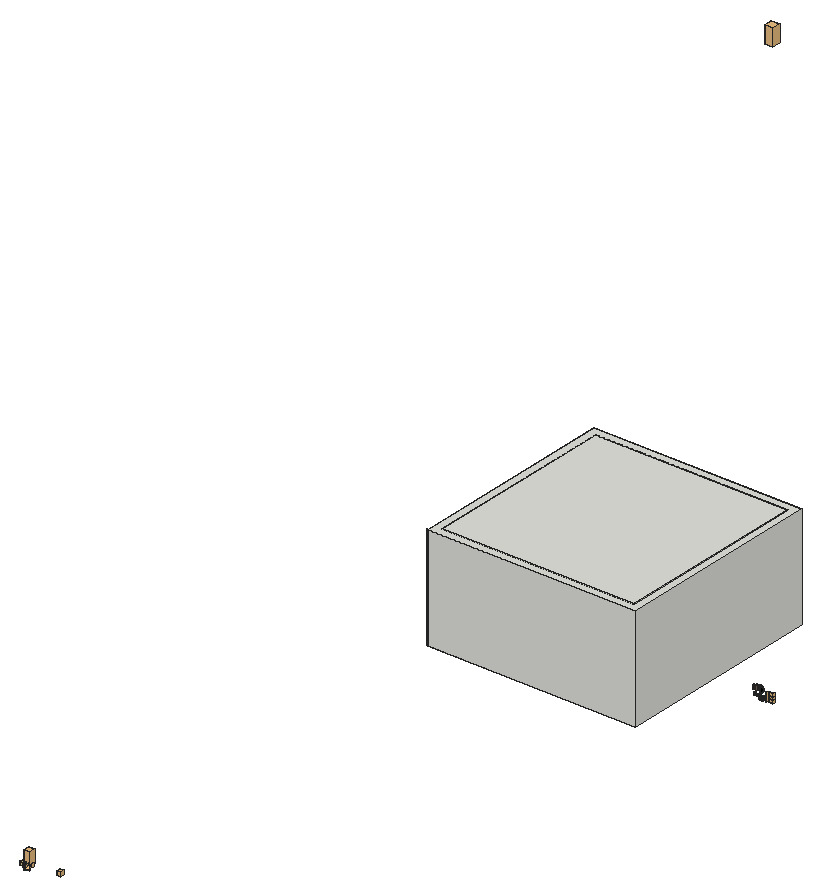
# SketchUp Ruby script. Lengths in inches.
U = 1.inch
M = Sketchup.active_model
def pt(a) = Geom::Point3d.new(a.map { |v| v * U })
def face(e, loops, mat)
  f = e.add_face(loops[0].map { |a| pt(a) })
  loops[1..].each { |l| e.add_face(l.map { |a| pt(a) }).erase! }
  f.material = f.back_material = mat if mat
  f
end
# faces: each face lists its corners as indices into pts; further lists are holes
def faces(e, pts, list, mat = nil) = list.each { |f| face(e, (f[0].is_a?(Array) ? f : [f]).map { |l| l.map { |i| pts[i] } }, mat) }
# xy, xz, yz: faces in a plane at the given z, y or x. An outline is a flat list of corners, or four numbers for a rectangle; further outlines are holes
def ring(l) = l.size == 4 ? [[l[0], l[1]], [l[2], l[1]], [l[2], l[3]], [l[0], l[3]]] : l.each_slice(2).to_a
def flat(e, list, mat, &to3) = list.each { |f| face(e, (f[0].is_a?(Array) ? f : [f]).map { |l| ring(l).map { |u, v| to3.(u, v) } }, mat) }
def xy(e, z, list, mat = nil) = flat(e, list, mat) { |x, y| [x, y, z] }
def xz(e, y, list, mat = nil) = flat(e, list, mat) { |x, z| [x, y, z] }
def yz(e, x, list, mat = nil) = flat(e, list, mat) { |y, z| [x, y, z] }
def lines(e, pts, list) = list.each { |a, b| e.add_line(pt(pts[a]), pt(pts[b])) }
# prism: a flat outline (further loops are holes) pulled along v
def prism(e, loops, v, mat = nil)
  f = face(e, loops, mat); d = Geom::Vector3d.new(v.map { |x| x * U })
  f.pushpull(f.normal.samedirection?(d) ? d.length : -d.length)
end
def box(e, o, s, mat = nil) = prism(e, [[o, [o[0] + s[0], o[1], o[2]], [o[0] + s[0], o[1] + s[1], o[2]], [o[0], o[1] + s[1], o[2]]]], [0, 0, s[2]], mat)
def at(x, y, z, deg = 0) = Geom::Transformation.translation(pt([x, y, z])) * Geom::Transformation.rotation(ORIGIN, Z_AXIS, deg.degrees)
def axes(o, x, y, z) = Geom::Transformation.new([*x, 0, *y, 0, *z, 0, *pt(o).to_a, 1])
def part(name) = M.definitions.add(name)
# library, detail: a bought-in or finely detailed component or shape, given as its bounding box
def library(name, o, s) = part(name).tap { |d| box(d.entities, o, s) }
def detail(e, o, s) = box(e.add_group.entities, o, s)
def put(e, d, t, mat = nil) = e.add_instance(d, t).tap { |i| i.material = mat if mat }
def group(e, t, mat = nil) = e.add_group.tap { |g| g.transformation = t; g.material = mat if mat }.entities
root = M.entities
M.materials.add("Lily_Light").color = [246, 247, 58]
M.materials.add("Polytec Natio Walnut").color = [132, 104, 79]
M.materials.add("SAMSUNG SMART FRIDGE").color = [78, 78, 81]
M.materials.add("[0045_Goldenrod]").color = [218, 165, 31]
M.materials["[0045_Goldenrod]"].alpha = 0.63
M.materials.add("[0066_Honeydew]").color = [240, 255, 240]
M.materials.add("[0130_Gainsboro]").color = [219, 219, 219]
M.materials.add("[0133_Gray]").color = [63, 63, 63]
M.materials.add("[Color M09]4").color = [0, 0, 0]
M.materials.add("[Translucent Glass Blue]").color = [100, 149, 237]
M.materials["[Translucent Glass Blue]"].alpha = 0.5
M.materials.add("cnwhc.com_草图联盟_1kmauOsh").color = [54, 52, 52]
M.materials.add("cnwhc.com_草图联盟_C8Y5Xp2O").color = [156, 156, 156]
M.materials["cnwhc.com_草图联盟_C8Y5Xp2O"].alpha = 0.15
M.materials.add("cnwhc.com_草图联盟_IHFcDxe1").color = [138, 151, 59]
M.materials.add("cnwhc.com_草图联盟_KNEfX85g").color = [162, 126, 87]
M.materials.add("cnwhc.com_草图联盟_QJow1Ky4").color = [144, 133, 65]
M.materials.add("cnwhc.com_草图联盟_z6N5x4Hv").color = [223, 205, 124]
c1 = part("Door Lever\#2")
detail(c1.entities,[0,0,0],[5.43,2.05,2.36])
c2 = part("Door Lever\#1")
detail(c2.entities,[0,0,0],[5.43,2.05,2.36])
c3 = part("Door Lever\#3")
detail(c3.entities,[0,0,0],[5.43,2.05,2.36])
c4 = part("200mm Half Round Handle")
xz(c4.entities,0,[[3.9375,0,3.9375,7.875,3.42,7.84,2.92,7.74,2.43,7.57,1.97,7.35,1.54,7.06,1.15,6.72,0.8125,6.33,0.53,5.91,0.3,5.44,0.13,4.96,0.03,4.45,0,3.9375,0.03,3.42,0.13,2.92,0.3,2.43,0.53,1.97,0.8125,1.54,1.15,1.15,1.54,0.8125,1.97,0.53,2.43,0.3,2.92,0.13,3.42,0.03]],"[Color M09]4")
xz(c4.entities,0.12,[[3.82,0.01,3.42,0.03,2.92,0.13,2.43,0.3,1.97,0.53,1.54,0.8125,1.15,1.15,0.8125,1.54,0.53,1.97,0.3,2.43,0.13,2.92,0.03,3.42,0,3.9375,0.03,4.45,0.13,4.96,0.3,5.44,0.53,5.91,0.8125,6.33,1.15,6.72,1.54,7.06,1.97,7.35,2.43,7.57,2.92,7.74,3.42,7.84,3.82,7.87]],"[Color M09]4")
xz(c4.entities,0.91,[[3.9375,0,3.82,0.01,3.82,7.87,3.9375,7.875]],"[Color M09]4")
yz(c4.entities,3.82,[[0.12,0.01,0.91,7.87]],"[Color M09]4")
yz(c4.entities,3.9375,[[0,0,0.91,7.875]],"[Color M09]4")
p = [[3.42,0,0.03],[2.92,0,0.13],[2.92,0.12,0.13],[3.42,0.12,0.03],[3.9375,0,0],[3.82,0.12,0.01],
  [3.82,0.91,0.01],[3.9375,0.91,0],[2.43,0,0.3],[2.43,0.12,0.3],[1.97,0,0.53],[1.97,0.12,0.53],
  [1.54,0,0.8125],[1.54,0.12,0.8125],[1.15,0,1.15],[1.15,0.12,1.15],[0.8125,0,1.54],[0.8125,0.12,1.54],
  [0.53,0,1.97],[0.53,0.12,1.97],[0.3,0,2.43],[0.3,0.12,2.43],[0.13,0,2.92],[0.13,0.12,2.92],
  [0.03,0,3.42],[0.03,0.12,3.42],[0,0,3.9375],[0,0.12,3.9375],[0.03,0,4.45],[0.03,0.12,4.45],
  [0.13,0,4.96],[0.13,0.12,4.96],[0.3,0,5.44],[0.3,0.12,5.44],[0.53,0,5.91],[0.53,0.12,5.91],
  [0.8125,0,6.33],[0.8125,0.12,6.33],[1.15,0,6.72],[1.15,0.12,6.72],[1.54,0,7.06],[1.54,0.12,7.06],
  [1.97,0,7.35],[1.97,0.12,7.35],[2.43,0,7.57],[2.43,0.12,7.57],[2.92,0,7.74],[2.92,0.12,7.74],
  [3.42,0,7.84],[3.42,0.12,7.84],[3.9375,0,7.875],[3.9375,0.91,7.875],[3.82,0.91,7.87],[3.82,0.12,7.87]]
faces(c4.entities,p,[[0,1,2,3],[4,0,3,5,6,7],[1,8,9,2],[8,10,11,9],[10,12,13,11],[12,14,15,13],[14,16,17,15],[16,18,19,17],
  [18,20,21,19],[20,22,23,21],[22,24,25,23],[24,26,27,25],[26,28,29,27],[28,30,31,29],[30,32,33,31],[32,34,35,33],
  [34,36,37,35],[36,38,39,37],[38,40,41,39],[40,42,43,41],[42,44,45,43],[44,46,47,45],[46,48,49,47],[48,50,51,52,53,49]],"[Color M09]4")
c5 = part("150mm Half Round Handle")
xz(c5.entities,0,[[0,0,0.12,0.01,0.12,5.9,0,5.91]],"Polytec Natio Walnut")
xz(c5.entities,0.79,[[0.12,0.01,0.39,0.03,0.76,0.1,1.13,0.22,1.48,0.4,1.8,0.61,2.09,0.86,2.34,1.16,2.56,1.48,2.73,1.82,2.85,2.1875,2.93,2.57,2.95,2.95,2.93,3.34,2.85,3.72,2.73,4.08,2.56,4.43,2.34,4.75,2.09,5.04,1.8,5.3,1.48,5.51,1.13,5.68,0.76,5.8,0.39,5.88,0.12,5.9]],"Polytec Natio Walnut")
xz(c5.entities,0.91,[[0,0,0,5.91,0.39,5.88,0.76,5.8,1.13,5.68,1.48,5.51,1.8,5.3,2.09,5.04,2.34,4.75,2.56,4.43,2.73,4.08,2.85,3.72,2.93,3.34,2.95,2.95,2.93,2.57,2.85,2.1875,2.73,1.82,2.56,1.48,2.34,1.16,2.09,0.86,1.8,0.61,1.48,0.4,1.13,0.22,0.76,0.1,0.39,0.03]],"Polytec Natio Walnut")
yz(c5.entities,0,[[0,0,0.91,5.91]],"Polytec Natio Walnut")
yz(c5.entities,0.12,[[0,0.01,0.79,5.9]],"Polytec Natio Walnut")
p = [[0,0.91,0],[0.39,0.91,0.03],[0.39,0.79,0.03],[0.12,0.79,0.01],[0.12,0,0.01],[0,0,0],
  [0.76,0.91,0.1],[0.76,0.79,0.1],[1.13,0.91,0.22],[1.13,0.79,0.22],[1.48,0.91,0.4],[1.48,0.79,0.4],
  [1.8,0.91,0.61],[1.8,0.79,0.61],[2.09,0.91,0.86],[2.09,0.79,0.86],[2.34,0.91,1.16],[2.34,0.79,1.16],
  [2.56,0.91,1.48],[2.56,0.79,1.48],[2.73,0.91,1.82],[2.73,0.79,1.82],[2.85,0.91,2.1875],[2.85,0.79,2.1875],
  [2.93,0.91,2.57],[2.93,0.79,2.57],[2.95,0.91,2.95],[2.95,0.79,2.95],[2.93,0.91,3.34],[2.93,0.79,3.34],
  [2.85,0.91,3.72],[2.85,0.79,3.72],[2.73,0.91,4.08],[2.73,0.79,4.08],[2.56,0.91,4.43],[2.56,0.79,4.43],
  [2.34,0.91,4.75],[2.34,0.79,4.75],[2.09,0.91,5.04],[2.09,0.79,5.04],[1.8,0.91,5.3],[1.8,0.79,5.3],
  [1.48,0.91,5.51],[1.48,0.79,5.51],[1.13,0.91,5.68],[1.13,0.79,5.68],[0.76,0.91,5.8],[0.76,0.79,5.8],
  [0.39,0.91,5.88],[0.39,0.79,5.88],[0,0.91,5.91],[0,0,5.91],[0.12,0,5.9],[0.12,0.79,5.9]]
faces(c5.entities,p,[[0,1,2,3,4,5],[1,6,7,2],[6,8,9,7],[8,10,11,9],[10,12,13,11],[12,14,15,13],[14,16,17,15],[16,18,19,17],
  [18,20,21,19],[20,22,23,21],[22,24,25,23],[24,26,27,25],[26,28,29,27],[28,30,31,29],[30,32,33,31],[32,34,35,33],
  [34,36,37,35],[36,38,39,37],[38,40,41,39],[40,42,43,41],[42,44,45,43],[44,46,47,45],[46,48,49,47],[48,50,51,52,53,49]],"Polytec Natio Walnut")
c6 = part("148mm Black Satin Pull\#1")
prism(c6.entities,[[[5.83,0.12,0.5],[5.83,0.16,0.49],[5.83,0.16,0],[5.83,0.31,0],[5.83,0.31,0.49],[5.83,0.35,0.5],[5.83,0.4,0.54],[5.83,0.44,0.59],[5.83,0.46,0.65],[5.83,0.47,0.71],[5.83,0.46,0.77],[5.83,0.44,0.83],[5.83,0.4,0.875],[5.83,0.35,0.91],[5.83,0.3,0.9375],[5.83,0.24,0.94],[5.83,0.18,0.9375],[5.83,0.12,0.91],[5.83,0.07,0.875],[5.83,0.03,0.83],[5.83,0.01,0.77],[5.83,0,0.71],[5.83,0.01,0.65],[5.83,0.03,0.59],[5.83,0.07,0.54]]],[-5.83,0,0],"[Color M09]4")
p = [[5.83,0.16,0.59],[0,0.16,0.59],[5.83,0.31,0.59],[0,0.31,0.59]]
lines(c6.entities,p,[[0,1],[2,3]])
c7 = part("232mm Slimline Handle\#1")
detail(c7.entities,[0,0,0],[9.13,0.47,1.38])
c8 = part("232mm Slimline Handle")
detail(c8.entities,[0,0,0],[9.13,0.47,1.38])
c9 = library("SAMSUNG SMART FRIDGE",[0,-0.09,0],[35.91,28.28,70.08])
c10 = library("Bosch Stove",[0,0,0],[36.22,20.12,1.38])
c11 = library("fff.dwg",[0.01,-0.93,0],[23.6,19.21,16.14])
c12 = part("Janela aluminio")
xy(c12.entities,0,[[0,0,47.24,1.57],[23.62,1.57,47.24,2.76],[0,2.76,25.98,3.9375],[0,3.9375,47.24,5.91]])
xy(c12.entities,43.31,[[0,0,47.24,1.57],[23.62,1.57,47.24,2.76],[0,2.76,0,5.91,47.24,5.91,47.24,3.9375,25.98,3.9375,25.98,2.76],[25.98,2.76,47.24,3.9375]])
xz(c12.entities,1.57,[[0,0,23.62,0,23.62,41.34,21.26,41.34,21.26,1.97,1.97,1.97,1.97,41.34,23.62,41.34,23.62,43.31,0,43.31],[[23.62,0,47.24,43.31],[25.7,1.97,45.28,41.34]]])
xz(c12.entities,2.76,[[[0,0,23.62,43.31],[2.36,2.36,21.26,40.94]],[23.62,0,25.98,43.31]])
xz(c12.entities,2.76,[[2.36,2.36,21.26,40.94]],"[Translucent Glass Blue]")
xz(c12.entities,3.9375,[[25.98,0,25.98,2.36,44.88,2.36,44.88,40.94,25.98,40.94,25.98,43.31,47.24,43.31,47.24,0]])
xz(c12.entities,3.9375,[[25.98,2.36,44.88,40.94]],"[Translucent Glass Blue]")
yz(c12.entities,0,[[0,0,1.57,43.31],[2.76,0,5.91,43.31]])
yz(c12.entities,23.62,[[1.57,0,2.76,43.31]])
yz(c12.entities,25.98,[[2.76,0,3.9375,43.31]])
yz(c12.entities,47.24,[[0,0,1.57,43.31],[1.57,0,2.76,43.31],[3.9375,0,5.91,43.31]])
c13 = library("Sink with faucet",[-0.11,0,0],[20.3,18.9,21.51])
c14 = library("Potted plant",[0.24,-1.94,0],[14.49,14.49,6.23])
c15 = library("KITCHEN+KNIFES",[-11.85,-0.97,-1.38],[30.4,24.23,12.79])
c16 = library("Micro+samsungCE170b-b+28L",[0.33,0.39,0],[20.66,20.36,12.2])
c17 = library("Lg+Water+purifier (1)",[0,2.4,0],[10.83,14.37,19.92])
c18 = library("Group8",[-17.72,-4.29,0],[35.44,8.58,13.65])
c19 = library("Group\#13",[-397.46,82.38,-0.11],[62.88,62.86,260])
c20 = library("Group\#10",[-282.65,82.375,-0.11],[62.85,62.875,260.02])
c21 = library("Group\#9",[222.96,189.98,-0.44],[259.48,39.25,337.49])
c22 = library("Group\#30",[41.52,-158.49,40.25],[95.93,90.14,172.87])
c23 = library("Group\#21",[-504.125,120.57,-0.1],[108.2,108.21,338.13])
c24 = library("Group\#22",[-376.9,120.94,-0.1],[107.79,107.8,326.37])
c25 = library("Group\#8",[-254.81,120.48,-0.6],[108.21,108.21,334.5])
c26 = library("Group\#24",[-133.01,121.19,-0.1],[106.95,106.95,324.89])
c27 = library("Group\#25",[0.46,121.12,-0.1],[106.94,106.94,338.14])
c28 = library("Group\#26",[151.35,137.54,-0.1],[70.51,70.14,256.45])
c29 = library("Group\#27",[-266.02,-201.27,40.23],[225.02,228.69,89.38])
c30 = library("Group\#7",[-78.56,-74.98,40.25],[131.28,107.59,245.3125])
c31 = library("Group\#31",[-60.55,-181.2,40.41],[105.85,106.35,65.49])
c32 = library("Group\#34",[253.59,42.68,151.97],[53.13,53.13,100.94])
c33 = library("Group\#35",[281.12,-5,151.97],[53.13,53.13,100.92])
c34 = library("Group\#6",[308.75,-52.85,151.97],[53.125,53.13,100.94])
c35 = library("Group\#4",[336.19,-100.38,151.98],[53.13,53.13,100.93])
c36 = library("Group\#3",[363.79,-148.1875,151.98],[53.13,53.13,100.93])
c37 = library("Group\#39",[253.59,42.68,30.7],[53.13,53.13,100.93])
c38 = library("Group\#40",[281.12,-5,30.7],[53.13,53.13,100.91])
c39 = library("Group\#41",[308.75,-52.85,30.7],[53.125,53.13,100.94])
c40 = library("Group\#42",[336.19,-100.38,30.7],[53.13,53.13,100.91])
c41 = library("Group\#43",[363.79,-148.1875,30.7],[53.13,53.13,100.93])
c42 = library("Group\#44",[212.54,-198.04,-0.24],[263.36,352.65,298.47])
c43 = library("Group\#29",[55.69,-19.19,40.37],[80.08,80.05,323.81])
c44 = library("Group\#53",[-462.66,84.21,613.65],[72.44,72.44,111.8])
c45 = library("Group\#55",[-457.8,68.7,378.69],[103.44,103.46,159.72])
c46 = library("Group\#54",[-210.76,89.58,378.69],[103.46,103.45,159.72])
c47 = library("Group\#56",[-332.7,68.71,378.69],[103.45,103.45,159.72])
c48 = library("Group\#52",[-374.05,84.21,613.65],[72.44,72.44,111.8])
c49 = library("Group\#51",[-289.4,84.22,613.65],[72.44,72.43,111.8])
c50 = library("Group\#50",[-198.8,84.74,613.85],[84,84,172.39])
c51 = library("Group\#49",[-105.26,84.74,613.85],[84,84,172.39])
c52 = library("Group\#47",[51.24,128.79,378.72],[113.79,95.47,197.69])
c53 = library("Group\#46",[179.9,72.7,378.72],[113.8,95.46,197.69])
c54 = library("Group\#45",[327.72,72.7,378.72],[113.79,95.46,197.69])
c55 = library("Group\#33",[309.63,77.04,613.73],[136.79,86.78,171.39])
c56 = library("Group\#32",[-15.73,84.74,613.85],[84,84,172.39])
c57 = library("Group\#12",[85.42,84.74,613.85],[84,84,172.42])
c58 = library("Group\#11",[193.57,84.74,613.85],[84,84,172.39])
c59 = library("Group\#79",[-453.95,-270.9,-0.08],[243.89,243.63,216.82])
c60 = library("Group\#59",[118.34,-437.05,68.8],[33.09,42.97,27.32])
c61 = library("Group\#60",[91.875,-459.8125,1.36],[84.84,84.82,167.94])
c62 = library("Group\#61",[93.63,-458.06,3.28],[81.33,81.31,90.04])
c63 = library("Group\#62",[114.46,-437.1875,150.05],[39.68,39.57,39.67])
c64 = library("Group\#63",[177.52,-496.26,3.28],[81.21,81.23,127.94])
c65 = library("Group\#64",[175.77,-498.01,1.36],[84.71,84.74,167.94])
c66 = library("Group\#65",[198.24,-475.92,149.53],[39.78,40.55,40.71])
c67 = library("Group\#66",[-248.47,-468.28,0.39],[392.05,393.05,278.56])
c68 = library("Group\#67",[-141.57,-278.65,11.2],[96.36,96.33,131.41])
c69 = library("Group\#68",[-62.08,-202.43,11.2],[96.04,96.07,131.41])
c70 = library("Group\#69",[18.13,-280.93,11.2],[96.51,96.54,131.41])
c71 = library("Group\#70",[-213.25,-366.61,11.2],[96.18,96.15,131.41])
c72 = library("Group\#71",[-61.03,-358.93,11.2],[96.54,96.51,131.41])
c73 = library("Group\#72",[8.05,-292.87,22.71],[116.19,111.01,218.49])
c74 = library("Group\#73",[-64.85,-368.89,23],[127.95,108.9,222.0625])
c75 = library("Group\#74",[-143.92,-281.53,22.82],[119.68,105.06,218.38])
c76 = library("Group\#75",[-64.19,-232.55,22.9],[102.65,128.29,224.14])
c77 = library("Group\#76",[-225.25,-376.69,19.19],[116.52,116.69,261.73])
c78 = library("Group\#77",[-138.35,-437.94,11.2],[96.49,96.52,131.41])
c79 = library("Group\#78",[-142.58,-458.38,19.87],[79.66,135.74,256])
c80 = library("Group\#134",[0,0,0],[4.57,4.57,4.5])
c81 = library("Group\#135",[-1.71,-2.49,0],[9.91,9.82,2.3125])
c82 = library("Group\#136",[-0.64,-0.9,0],[7.41,7.04,15.0625])
c83 = library("Group\#133",[0,0,0],[4.57,4.57,8.43])
c84 = library("Group\#151",[-1.45,-1.88,0],[9.58,9.75,16.01])
c85 = library("Group\#176",[0,0,0],[4.57,4.57,4.68])
xy(root,0,[[[1,0,241,240],[170.43,22,170.43,33,32,33,32,231,232,231,232,22]],[173.43,22,232,22,232,231,32,231,32,33,171.43,33,171.43,37,173.43,37],[170.43,22,173.43,22,173.43,36,171.43,36,171.43,33,170.43,33]])
xy(root,1,[[32,33,33,231],[33,33,170.43,34],[170.43,33,171.43,34]])
xy(root,4,[[170.43,22,171.43,34],[33,34,33,231,34,231,34,200.75,33.6,200.75,33.6,199.75,34,199.75,34,170,33.6,170,33.6,169,34,169,34,139.25,33.6,139.25,33.6,138.25,34,138.25,34,49,33.6,49,33.6,47,34,47,34,34],[34,34,34,36,123.43,36,123.43,35,124.43,35,124.43,36,146.93,36,146.93,35,147.93,35,147.93,36,171.43,36,171.43,34],[146.93,35,147.93,35.4]])
xy(root,14.15,[[58,35,58.08,35.6],[58.08,35,123.43,35.6],[58,35.6,58.08,36],[58.08,35.6,123.43,36],[33,60,34,108]])
xy(root,15.15,[[58,35,123.43,35.6],[58,35.6,123.43,36],[33,60,34,108]])
xy(root,21.3125,[[12,38,32,58]])
xy(root,24.79,[[58,35,58.08,35.6],[58.08,35,123.43,35.6],[58,35.6,58.08,36],[58.08,35.6,123.43,36],[33,60,34,108]])
xy(root,25.79,[[58,35,123.43,35.6],[58,35.6,123.43,37],[33,60,34,108]])
xy(root,35.9375,[[34,22,34,36,58,36,58,37,123.43,37,123.43,35,124.43,35,124.43,36,146.93,36,146.93,35,147.93,35,147.93,36,171.43,36,171.43,22],[171.43,22,172.43,36],[123.43,35,124.43,35,124.43,36,146.93,36,146.93,35.4,147.43,35.4,147.43,37,123.43,37],[146.93,35,147.43,35.4],[147.43,35,147.93,35.4],
  [147.43,35.4,147.93,35.4,147.93,36,171.43,36,171.43,37,147.43,37],[34,36,58,37],[171.43,36,172.43,37],[34,37,34,47,33.6,47,33.6,49,34,49,34,58,35,58,35,37],[34,58,34,138.25,33.6,138.25,33.6,139.25,34,139.25,34,169,33.6,169,33.6,170,34,170,34,199.75,33.6,199.75,33.6,200.75,34,200.75,34,231,35,231,35,58]])
xy(root,37.9375,[[[10,22,171.43,22,171.43,37,35,37,35,231,10,231],[12,38,32,58]],[171.43,22,172.43,36],[171.43,36,172.43,37]])
xy(root,48,[[1,33,10,69]])
xy(root,49,[[147.43,22,171.43,26]])
xy(root,49.5,[[147.93,14,170.93,26]])
xy(root,51.9375,[[10,22,87.43,25.6]])
xy(root,54.4375,[[12.5,9,46.21,25.6],[51.21,9,84.93,25.6]])
xy(root,62.17,[[[147.93,14,170.93,26],[148.48,14.76,169.79,16.51]],[123.43,22,146.43,26]])
xy(root,62.17,[[148.48,14.76,169.79,16.51]],"Lily_Light")
xy(root,63.17,[[147.93,14,170.93,26]])
xy(root,64.17,[[125.43,14,144.43,26]])
xy(root,64.79,[[[12.5,9,46.21,25.6],[16.66,11.93,39.98,15.81]],[[51.21,9,84.93,25.6],[52.86,11.41,76.17,15.29]]])
xy(root,64.79,[[52.86,11.41,76.17,15.29],[16.66,11.93,39.98,15.81]],"Lily_Light")
xy(root,65.79,[[51.21,8.125,84.93,25.6],[12.5,9,46.21,25.6]])
xy(root,72,[[175.1875,22,175.1875,26,202.59,26,202.59,25.6,204.59,25.6,204.59,26,232,26,232,22]])
xy(root,75.08,[[125.43,14,125.43,17.87,142.64,17.87,142.64,18.87,125.43,18.87,125.43,26,144.43,26,144.43,14]])
xy(root,75.08,[[125.43,17.87,142.64,18.87]],"Lily_Light")
xy(root,75.83,[[[147.93,14,170.93,26],[148.48,14.76,169.79,16.51]]])
xy(root,75.83,[[148.48,14.76,169.79,16.51]],"Lily_Light")
xy(root,76.15,[[[51.21,8.125,84.93,25.6],[52.86,11.41,76.17,15.29]],[[12.5,9,46.21,25.6],[15.42,11.41,38.73,15.29]]])
xy(root,76.15,[[15.42,11.41,38.73,15.29],[52.86,11.41,76.17,15.29]],"Lily_Light")
xy(root,76.83,[[147.93,14,170.93,26]])
xy(root,77.08,[[125.43,17,144.43,26]])
xy(root,77.15,[[12.5,9,46.21,25.6],[51.21,9,84.93,25.6]])
xy(root,84,[[1,33,10,69]])
xy(root,87.5,[[[12.5,9,46.21,25.6],[15.42,11.41,38.73,15.29]],[[51.21,9,84.93,25.6],[52.86,11.41,76.17,15.29]]])
xy(root,87.5,[[15.42,11.41,38.73,15.29],[52.86,11.41,76.17,15.29]],"Lily_Light")
xy(root,88,[[125.43,17,125.43,17.87,142.64,17.87,142.64,18.87,125.43,18.87,125.43,26,144.14,26,144.14,17],[144.14,17,144.43,26],[175.1875,22,232,22,232,26,204.59,26,204.59,25.6,202.59,25.6,202.59,26,175.1875,26]])
xy(root,88,[[125.43,17.87,142.64,18.87]],"Lily_Light")
xy(root,89.5,[[[147.93,14,170.93,26],[148.48,14.76,169.79,16.51]],[171.43,25.6,173.43,37]])
xy(root,89.5,[[148.48,14.76,169.79,16.51]],"Lily_Light")
xy(root,90,[[87.43,22,87.43,25.6,86.57,25.6,86.57,26,113.86,26,113.86,25.6,115.86,25.6,115.86,26,123.43,26,123.43,22],[146.43,22,147.43,26],[171.43,22,173.43,25.6],[173.43,22,173.43,26,201.71,26,201.71,25.6,203.71,25.6,203.71,26,232,26,232,22],[10,25.6,10,231,27,231,27,191,26.6,191,26.6,189,27,189,27,150,26.6,150,26.6,148,27,148,27,109,26.6,109,26.6,107,27,107,27,68,26.6,68,26.6,66,27,66,27,26,55.29,26,55.29,25.6],
  [57.29,25.6,84.57,26],[143.14,25.6,145.14,26]])
xy(root,108,[[10,9,232,9,232,26,203.71,26,203.71,25.6,201.71,25.6,201.71,26,173.43,26,173.43,25.6,171.43,25.6,171.43,26,145.14,26,145.14,25.6,143.14,25.6,143.14,26,115.86,26,115.86,25.6,113.86,25.6,113.86,26,86.57,26,86.57,25.6,84.57,25.6,84.57,26,57.29,26,57.29,25.6,55.29,25.6,55.29,26,27,26,27,66,26.6,66,26.6,68,27,68,27,107,26.6,107,26.6,109,27,109,27,148,26.6,148,26.6,150,27,150,27,189,26.6,189,26.6,191,27,191,27,231,10,231]])
xy(root,120,[[[1,0,241,240],[10,9,232,231]]])
xz(root,0,[[0,0,1,120],[1,0,240,120],[240,0,241,120]])
xz(root,8.125,[[51.21,65.79,84.93,76.15]])
xz(root,9,[[12.5,54.4375,46.21,64.79],[51.21,54.4375,84.93,64.79],[12.5,65.79,46.21,76.15],[12.5,77.15,46.21,87.5],[51.21,77.15,84.93,87.5],
  [10,108,232,120]])
xz(root,14,[[147.93,49.5,170.93,62.17],[147.93,63.17,170.93,75.83],[125.43,64.17,144.43,75.08],[147.93,76.83,170.93,89.5]])
xz(root,17,[[125.43,77.08,144.43,88]])
xz(root,22,[[170.43,0,173.43,0,173.43,90,171.43,90,171.43,37.9375,172.43,37.9375,172.43,35.9375,171.43,35.9375,171.43,4,170.43,4],[173.43,0,173.43,90,232,90,232,88,175.1875,88,175.1875,72,232,72,232,0],[10,35.9375,34,37.9375],[34,35.9375,172.43,37.9375],[10,37.9375,10,51.9375,87.43,51.9375,87.43,90,123.43,90,123.43,62.17,146.43,62.17,146.43,90,147.43,90,147.43,49,171.43,49,171.43,37.9375]])
xz(root,25.6,[[[10,51.9375,87.43,90],[12.5,54.4375,84.93,87.5]],[46.21,54.4375,48.71,87.5],[48.71,54.4375,51.21,87.5],[12.5,64.79,46.21,65.79],[51.21,64.79,84.93,65.79],
  [202.59,72,204.59,88],[12.5,76.15,46.21,77.15],[51.21,76.15,84.93,77.15],[171.43,89.5,173.43,90],[55.29,90,57.29,108],
  [84.57,90,86.57,108],[113.86,90,115.86,108],[143.14,90,145.14,108],[171.43,90,173.43,108],[201.71,90,203.71,108]])
xz(root,25.6,[[12.5,54.4375,46.21,64.79],[51.21,54.4375,84.93,64.79],[12.5,65.79,46.21,76.15],[51.21,65.79,84.93,76.15],[12.5,77.15,46.21,87.5],
  [51.21,77.15,84.93,87.5]],"[Translucent Glass Blue]")
xz(root,26,[[[147.43,49,171.43,90],[147.93,49.5,170.93,89.5]],[[123.43,62.17,146.43,90],[125.43,64.17,144.43,88]],[147.93,62.17,170.93,63.17],[175.1875,72,202.59,88],[204.59,72,232,88],
  [125.43,75.08,144.43,77.08],[147.93,75.83,170.93,76.83],[27,90,55.29,108],[57.29,90,84.57,108],[86.57,90,113.86,108],
  [115.86,90,143.14,108],[145.14,90,171.43,108],[173.43,90,201.71,108],[203.71,90,232,108]])
xz(root,26,[[147.93,49.5,170.93,62.17],[147.93,63.17,170.93,75.83],[125.43,64.17,144.43,75.08],[147.93,76.83,170.93,89.5],[125.43,77.08,144.43,88]],"[Translucent Glass Blue]")
xz(root,33,[[1,48,10,84]])
xz(root,33,[[32,0,171.43,1]],"Lily_Light")
xz(root,34,[[33,1,171.43,4]])
xz(root,35,[[123.43,4,124.43,35.9375],[58,14.15,123.43,15.15],[58,24.79,123.43,25.79]])
xz(root,35.4,[[146.93,4,147.93,35.9375]])
xz(root,35.6,[[58,14.15,123.43,15.15],[58,24.79,123.43,25.79]])
xz(root,36,[[34,4,58,35.9375],[58,4,123.43,14.15],[124.43,4,146.93,35.9375],[147.93,4,171.43,35.9375],[58,15.15,123.43,24.79]])
xz(root,37,[[171.43,0,171.43,35.9375,172.43,35.9375,172.43,37.9375,171.43,37.9375,171.43,89.5,173.43,89.5,173.43,0],[58,25.79,123.43,35.9375],[35,35.9375,58,37.9375],[58,35.9375,172.43,37.9375]])
xz(root,38,[[12,21.3125,32,37.9375]])
xz(root,47,[[33.6,4,34,35.9375]])
xz(root,49,[[33.6,4,34,35.9375]])
xz(root,58,[[12,21.3125,32,37.9375]])
xz(root,60,[[33,14.15,34,15.15],[33,24.79,34,25.79]])
xz(root,66,[[26.6,90,27,108]])
xz(root,68,[[26.6,90,27,108]])
xz(root,69,[[1,48,10,84]])
xz(root,107,[[26.6,90,27,108]])
xz(root,108,[[33,14.15,34,15.15],[33,24.79,34,25.79]])
xz(root,109,[[26.6,90,27,108]])
xz(root,138.25,[[33.6,4,34,35.77],[33.6,35.77,34,35.9375]])
xz(root,139.25,[[33.6,4,34,35.77],[33.6,35.77,34,35.9375]])
xz(root,148,[[26.6,90,27,108]])
xz(root,150,[[26.6,90,27,108]])
xz(root,169,[[33.6,4,34,35.82],[33.6,35.82,34,35.9375]])
xz(root,170,[[33.6,4,34,35.82],[33.6,35.82,34,35.9375]])
xz(root,189,[[26.6,90,27,108]])
xz(root,191,[[26.6,90,27,108]])
xz(root,199.75,[[33.6,4,34,35.88],[33.6,35.88,34,35.9375]])
xz(root,200.75,[[33.6,4,34,35.88],[33.6,35.88,34,35.9375]])
xz(root,231,[[32,0,232,0,232,120,10,120,10,108,27,108,27,90,10,90,10,37.9375,35,37.9375,35,35.9375,34,35.9375,34,4,33,4,33,1,32,1],[10,35.9375,35,37.9375]])
xz(root,240,[[1,0,241,120]])
yz(root,1,[[[0,0,240,120],[33,48,69,84]]])
yz(root,10,[[22,35.9375,58,37.9375],[58,35.9375,231,37.9375],[[22,37.9375,231,37.9375,231,90,25.6,90,25.6,51.9375,22,51.9375],[33,48,69,84]],[9,108,231,120]])
yz(root,12,[[38,21.3125,58,37.9375]])
yz(root,12.5,[[9,54.4375,25.6,64.79],[9,65.79,25.6,76.15],[9,77.15,25.6,87.5]])
yz(root,26.6,[[66,90,68,108],[107,90,109,108],[148,90,150,108],[189,90,191,108]])
yz(root,27,[[26,90,66,108],[68,90,107,108],[109,90,148,108],[150,90,189,108],[191,90,231,108],
  [231,90,232,108]])
yz(root,32,[[38,21.3125,47.5,23.9375],[47.5,21.3125,48.5,37.9375],[48.5,21.3125,58,23.9375],[38,23.9375,47.5,37.9375],[48.5,23.9375,58,37.9375]])
yz(root,32,[[33,0,231,1]],"Lily_Light")
yz(root,33,[[34,1,231,4],[60,14.15,108,15.15],[60,24.79,108,25.79]])
yz(root,33.6,[[47,4,49,35.9375],[138.25,4,139.25,35.9375],[169,4,170,35.9375],[199.75,4,200.75,35.9375]])
yz(root,34,[[36,4,47,35.9375],[49,4,60,35.9375],[60,4,108,14.15],[108,4,138.25,35.9375],[139.25,4,169,35.9375],
  [170,4,199.75,35.9375],[200.75,4,231,35.9375],[60,15.15,108,24.79],[60,25.79,108,35.9375]])
yz(root,35,[[37,35.9375,231,37.9375]])
yz(root,46.21,[[9,54.4375,25.6,64.79],[9,65.79,25.6,76.15],[9,77.15,25.6,87.5]])
yz(root,51.21,[[9,54.4375,25.6,64.79],[8.125,65.79,25.6,76.15],[9,77.15,25.6,87.5]])
yz(root,55.29,[[25.6,90,26,108]])
yz(root,57.29,[[25.6,90,26,108]])
yz(root,58,[[35,14.15,35.6,15.15],[35.6,14.15,36,15.15],[35,24.79,35.6,25.79],[35.6,24.79,36,25.79],[36,25.79,37,35.9375]])
yz(root,84.57,[[25.6,90,26,108]])
yz(root,84.93,[[9,54.4375,25.6,64.79],[8.125,65.79,25.6,76.15],[9,77.15,25.6,87.5]])
yz(root,86.57,[[25.6,90,26,108]])
yz(root,87.43,[[22,51.9375,25.6,90]])
yz(root,113.86,[[25.6,90,26,108]])
yz(root,115.86,[[25.6,90,26,108]])
yz(root,123.43,[[35,4,36,14.15],[35,14.15,35.6,15.15],[35,15.15,36,24.79],[35,24.79,35.6,25.79],[35,25.79,37,35.9375],
  [22,62.17,26,90]])
yz(root,124.43,[[35,4,36,35.9375]])
yz(root,125.43,[[14,64.17,26,75.08],[17,77.08,26,88]])
yz(root,143.14,[[25.6,90,26,108]])
yz(root,144.43,[[14,64.17,26,75.08],[17,77.08,26,88]])
yz(root,145.14,[[25.6,90,26,108]])
yz(root,146.43,[[22,62.17,26,90]])
yz(root,146.93,[[35,4,35.4,35.9375],[35.4,4,36,35.9375]])
yz(root,147.43,[[22,49,26,90]])
yz(root,147.93,[[35,4,35.4,35.9375],[35.4,4,36,35.9375],[14,49.5,26,62.17],[14,63.17,26,75.83],[14,76.83,26,89.5]])
yz(root,170.93,[[14,49.5,26,62.17],[14,63.17,26,75.83],[14,76.83,26,89.5]])
yz(root,171.43,[[33,0,33,1,34,1,34,4,36,4,36,35.9375,37,35.9375,37,0],[22,4,36,35.9375],[22,37.9375,22,49,26,49,26,89.5,37,89.5,37,37.9375],[22,49,26,49,26,89.5,25.6,89.5,25.6,90,22,90],[25.6,89.5,26,108]])
yz(root,172.43,[[22,35.9375,36,37.9375],[36,35.9375,37,37.9375]])
yz(root,173.43,[[22,0,36,0,36,89.5,25.6,89.5,25.6,90,22,90],[36,0,37,89.5],[25.6,89.5,26,90],[25.6,90,26,108]])
yz(root,175.1875,[[22,72,26,88]])
yz(root,201.71,[[25.6,90,26,108]])
yz(root,202.59,[[25.6,72,26,88]])
yz(root,203.71,[[25.6,90,26,108]])
yz(root,204.59,[[25.6,72,26,88]])
yz(root,232,[[22,0,22,72,26,72,26,88,22,88,22,90,26,90,26,108,9,108,9,120,231,120,231,0]])
yz(root,241,[[0,0,240,120]])
p = [[12,58,35.9375],[10,58,35.9375],[32,58,35.9375],[34,58,35.9375],[123.43,36,24.79],[123.51,36,24.79],
  [34,200.25,3.94],[34,200.25,4],[34,169.5,3.89],[34,169.5,4],[34,138.75,3.83],[34,138.75,4],
  [34,108,3.77],[34,108,4],[173.43,36,90],[173.43,36,89.5]]
lines(root,p,[[0,1],[2,3],[4,5],[6,7],[8,9],[10,11],[12,13],[14,15]])
put(root,c1,axes([358.29,47.21,57.2],[1,0,0],[0,-1,0],[0,0,-1]))
put(root,c2,axes([358.29,47.21,50],[1,0,0],[0,-1,0],[0,0,-1]))
put(root,c3,axes([358.29,47.21,53.6],[1,0,0],[0,-1,0],[0,0,-1]))
put(root,c4,at(352.17,46.06,53.16,-180))
put(root,c5,at(343.85,45.16,54.39))
put(root,c6,axes([350.39,45.16,46.41],[1,0,0],[0,0,-1],[0,1,0]))
put(root,c7,axes([201.21,26,84.27],[0,0,-1],[-1,0,0],[0,1,0]),"[Color M09]4")
put(root,c8,axes([356.15,45.16,56.46],[0,0,-1],[-1,0,0],[0,1,0]),"[Color M09]4")
put(root,c7,axes([205.74,26,84.39],[0,0,-1],[-1,0,0],[0,1,0]),"[Color M09]4")
put(root,c7,axes([205.74,26,101.95],[0,0,-1],[-1,0,0],[0,1,0]),"[Color M09]4")
put(root,c7,axes([200.07,26,102.05],[0,0,-1],[-1,0,0],[0,1,0]),"[Color M09]4")
put(root,c7,axes([146.82,26,102.05],[0,0,-1],[-1,0,0],[0,1,0]),"[Color M09]4")
put(root,c7,axes([141.76,26,102.05],[0,0,-1],[-1,0,0],[0,1,0]),"Lily_Light")
put(root,c7,axes([89.13,26,102.05],[0,0,-1],[-1,0,0],[0,1,0]),"[Color M09]4")
put(root,c7,axes([82.82,26,102.05],[0,0,-1],[-1,0,0],[0,1,0]))
put(root,c7,axes([52.63,26,102.05],[0,0,-1],[-1,0,0],[0,1,0]),"[Color M09]4")
put(root,c7,axes([27,69.48,92.88],[0,0,1],[0,-1,0],[1,0,0]),"[Color M09]4")
put(root,c7,axes([27,64.54,92.88],[0,0,1],[0,-1,0],[1,0,0]),"[Color M09]4")
put(root,c7,axes([27,111.04,92.88],[0,0,1],[0,-1,0],[1,0,0]),"[Color M09]4")
put(root,c7,axes([27,192.29,92.88],[0,0,1],[0,-1,0],[1,0,0]),"[Color M09]4")
put(root,c7,axes([27,187.48,92.88],[0,0,1],[0,-1,0],[1,0,0]),"[Color M09]4")
put(root,c7,axes([34,50.53,16.41],[0,0,1],[0,-1,0],[1,0,0]),"[Color M09]4")
put(root,c7,axes([34,45.96,16.41],[0,0,1],[0,-1,0],[1,0,0]),"[Color M09]4")
put(root,c7,axes([34,79.93,9.96],[0,1,0],[0,0,1],[1,0,0]),"[Color M09]4")
put(root,c7,axes([34,79.93,20.83],[0,1,0],[0,0,1],[1,0,0]),"[Color M09]4")
put(root,c7,axes([34,141.23,17.53],[0,0,1],[0,-1,0],[1,0,0]))
put(root,c7,axes([34,137.23,17.53],[0,0,1],[0,-1,0],[1,0,0]),"[Color M09]4")
put(root,c7,axes([34,198.04,17.53],[0,0,1],[0,-1,0],[1,0,0]),"[Color M09]4")
put(root,c7,axes([34,202.67,17.53],[0,0,1],[0,-1,0],[1,0,0]),"[Color M09]4")
put(root,c7,axes([149.41,36,25.58],[0,0,-1],[-1,0,0],[0,1,0]))
put(root,c7,axes([145.79,36,25.58],[0,0,-1],[-1,0,0],[0,1,0]))
put(root,c7,axes([54.79,36,25.58],[0,0,-1],[-1,0,0],[0,1,0]),"[Color M09]4")
put(root,c7,axes([95.34,36,19.69],[-1,0,0],[0,0,1],[0,1,0]),"[Color M09]4")
put(root,c7,axes([95.22,36,31.25],[-1,0,0],[0,0,1],[0,1,0]),"[Color M09]4")
put(root,c7,axes([95.53,36,9.13],[-1,0,0],[0,0,1],[0,1,0]),"[Color M09]4")
put(root,c9,axes([219.7,46.93,0],[-0.9384,0,0],[0,-1,0],[0,0,0.92]))
put(root,c10,axes([85.24,22,39.1],[0.99,0,0],[0,0.7644,0],[0,0,1]))
put(root,c11,axes([113.5,22,71.72],[-1,0,0],[0,0,1],[0,0.8,0]))
put(root,c12,axes([4.66,33,48],[0,0.762,0],[-0.62,0,0],[0,0,0.83127]))
put(root,c13,axes([10.12,37.52,29.8125],[1.09852,0,0],[0,1.14,0],[0,0,0.84]))
put(root,c14,axes([154.11,15.5,76.83],[0.5,0,0],[0,0.5,0],[0,0,0.58195]))
put(root,c14,axes([4.51,36.64,48],[0.305,0,0],[0,0.305,0],[0,0,0.46504]))
put(root,c14,axes([154.11,15.5,49.375],[0.5,0,0],[0,0.5,0],[0,0,0.58195]))
put(root,c15,axes([44.2,24.21,38.81],[0.57596,0,0],[0,0.57596,0],[0,0,0.57596]))
put(root,c14,axes([12.78,24.68,37.9375],[0.305,0,0],[0,0.305,0],[0,0,0.35499]))
put(root,c16,at(12.31,133.58,37.9375))
put(root,c17,at(10,176.57,50.41))
g1 = group(root,at(346.72,46.58,46.43))
prism(g1,[[[2.36,-0.48,-0.13],[2.36,-0.5,-0.18],[2.36,-1.42,-0.18],[2.36,-1.42,-0.33],[2.36,-0.5,-0.33],[2.36,-0.48,-0.38],[2.36,-0.4375,-0.4375],[2.36,-0.38,-0.48],[2.36,-0.32,-0.5],[2.36,-0.26,-0.51],[2.36,-0.19,-0.5],[2.36,-0.13,-0.48],[2.36,-0.07,-0.4375],[2.36,-0.03,-0.38],[2.36,-0.01,-0.32],[2.36,0,-0.26],[2.36,-0.01,-0.19],[2.36,-0.03,-0.13],[2.36,-0.07,-0.07],[2.36,-0.13,-0.03],[2.36,-0.19,-0.01],[2.36,-0.26,0],[2.36,-0.32,-0.01],[2.36,-0.38,-0.03],[2.36,-0.4375,-0.07]]],[-2.36,0,0])
g2 = group(root,at(341.34,45.91,49.28))
detail(g2,[0,-0.75,-1.1],[11.18,0.75,1.1])
g3 = group(root,at(340.82,46.34,59.02))
detail(g3,[0,-1.18,-1.58],[1.58,1.18,1.58])
g4 = group(root,at(341.34,45.91,51.54))
detail(g4,[0,-0.75,-1.1],[11.18,0.75,1.1])
g5 = group(root,at(340.82,46.34,56.3))
detail(g5,[0,-1.18,-1.58],[1.58,1.18,1.58])
put(root,c18,axes([134.04,21.34,64.17],[0.39508,0,0],[0,0.5057,0],[0,0,0.53336]))
put(root,c19,axes([20.05,90.36,44.97],[0.00191,0,0],[0,0.00191,0],[0,0,0.00191]))
put(root,c20,axes([20.05,90.36,44.97],[0.00191,0,0],[0,0.00191,0],[0,0,0.00191]))
put(root,c21,axes([20.05,90.36,44.97],[0.00191,0,0],[0,0.00191,0],[0,0,0.00191]))
put(root,c22,axes([127.14,36.39,35.53],[0.0598,0,0],[0,0.0598,0],[0,0,0.0598]))
put(root,c23,axes([20.05,90.36,44.97],[0.00191,0,0],[0,0.00191,0],[0,0,0.00191]))
put(root,c24,axes([20.05,90.36,44.97],[0.00191,0,0],[0,0.00191,0],[0,0,0.00191]))
put(root,c25,axes([20.05,90.36,44.97],[0.00191,0,0],[0,0.00191,0],[0,0,0.00191]))
put(root,c26,axes([20.05,90.36,44.97],[0.00191,0,0],[0,0.00191,0],[0,0,0.00191]))
put(root,c27,axes([20.05,90.36,44.97],[0.00191,0,0],[0,0.00191,0],[0,0,0.00191]))
put(root,c28,axes([65.04,20.59,37.94],[0.04365,0,0],[0,0.04365,0],[0,0,0.04365]))
put(root,c29,axes([20.05,90.36,44.89],[0.00191,0,0],[0,0.00191,0],[0,0,0.00191]))
put(root,c30,axes([144.81,31.62,36.2],[0.04306,0,0],[0,0.04306,0],[0,0,0.04306]))
put(root,c31,axes([20.05,90.36,44.89],[0.00191,0,0],[0,0.00191,0],[0,0,0.00191]))
put(root,c32,axes([20.05,90.36,44.97],[0.00191,0,0],[0,0.00191,0],[0,0,0.00191]))
put(root,c33,axes([20.05,90.36,44.97],[0.00191,0,0],[0,0.00191,0],[0,0,0.00191]))
put(root,c34,axes([20.05,90.36,44.97],[0.00191,0,0],[0,0.00191,0],[0,0,0.00191]))
put(root,c35,axes([20.05,90.36,44.97],[0.00191,0,0],[0,0.00191,0],[0,0,0.00191]))
put(root,c36,axes([20.05,90.36,44.97],[0.00191,0,0],[0,0.00191,0],[0,0,0.00191]))
put(root,c37,axes([20.05,90.36,44.97],[0.00191,0,0],[0,0.00191,0],[0,0,0.00191]))
put(root,c38,axes([20.05,90.36,44.97],[0.00191,0,0],[0,0.00191,0],[0,0,0.00191]))
put(root,c39,axes([20.05,90.36,44.97],[0.00191,0,0],[0,0.00191,0],[0,0,0.00191]))
put(root,c40,axes([20.05,90.36,44.97],[0.00191,0,0],[0,0.00191,0],[0,0,0.00191]))
put(root,c41,axes([20.05,90.36,44.97],[0.00191,0,0],[0,0.00191,0],[0,0,0.00191]))
put(root,c42,axes([20.05,90.36,44.97],[0.00191,0,0],[0,0.00191,0],[0,0,0.00191]))
put(root,c43,axes([134.98,30.55,36.34],[0.03947,0,0],[0,0.03947,0],[0,0,0.03947]))
put(root,c23,axes([72.94,16.26,77.15],[0.03014,0,0],[0,0.03014,0],[0,0,0.03014]))
put(root,c25,axes([72.94,16.26,77.15],[0.03014,0,0],[0,0.03014,0],[0,0,0.03014]))
put(root,c26,axes([72.94,16.26,77.15],[0.03014,0,0],[0,0.03014,0],[0,0,0.03014]))
put(root,c27,axes([72.94,16.26,77.15],[0.03014,0,0],[0,0.03014,0],[0,0,0.03014]))
put(root,c24,axes([72.94,16.26,77.15],[0.03014,0,0],[0,0.03014,0],[0,0,0.03014]))
put(root,c44,axes([37.91,28.53,14.25],[-0.08395,0,0],[0,-0.08395,0],[0,0,0.08395]))
put(root,c45,axes([1.92,27.21,45.76],[-0.05289,0,0],[0,-0.05289,0],[0,0,0.05289]))
put(root,c46,axes([31.91,26.3,48.85],[-0.04471,0,0],[0,-0.04471,0],[0,0,0.04471]))
put(root,c47,axes([16.18,29.55,44.02],[-0.0575,0,0],[0,-0.0575,0],[0,0,0.0575]))
put(root,c48,axes([37.91,26.59,14.25],[-0.08395,0,0],[0,-0.08395,0],[0,0,0.08395]))
put(root,c49,axes([37.91,28.46,14.25],[-0.08395,0,0],[0,-0.08395,0],[0,0,0.08395]))
put(root,c50,axes([63.33,26.21,24.75],[-0.05893,0,0],[0,-0.0483,0],[0,0,0.0483]))
put(root,c51,axes([63.33,26.21,24.75],[-0.05893,0,0],[0,-0.0483,0],[0,0,0.0483]))
put(root,c52,axes([41.37,26.28,68.83],[-0.02403,0,0],[0,-0.0383,0],[0,0,0.02314]))
put(root,c53,axes([33.32,24.68,39.19],[-0.04025,0,0],[0,-0.04025,0],[0,0,0.04025]))
put(root,c54,axes([57.22,26.45,37.43],[-0.0449,0,0],[0,-0.0449,0],[0,0,0.0449]))
put(root,c55,axes([44.38,25.28,50.33],[-0.0437,0,0],[0,-0.0437,0],[0,0,0.0437]))
put(root,c56,axes([63.33,26.21,24.75],[-0.05893,0,0],[0,-0.0483,0],[0,0,0.0483]))
put(root,c57,axes([-4.47,536.55,315.91],[-0.115,0,0],[0,-0.115,0],[0,0,0.115]))
put(root,c58,axes([44.38,25.28,50.33],[-0.0437,0,0],[0,-0.0437,0],[0,0,0.0437]))
put(root,c54,axes([48.9,26.45,37.43],[-0.0449,0,0],[0,-0.0449,0],[0,0,0.0449]))
put(root,c59,axes([145.04,26.68,77.08],[0.02951,0,0],[0,0.03574,0],[0,0,0.01926]))
put(root,c60,axes([24.28,93.18,37.93],[0.03192,0,0],[0,0.03192,0],[0,0,0.03192]),"cnwhc.com_草图联盟_IHFcDxe1")
put(root,c61,axes([24.28,93.18,37.93],[0.03192,0,0],[0,0.03192,0],[0,0,0.03192]),"cnwhc.com_草图联盟_C8Y5Xp2O")
put(root,c62,axes([24.28,93.18,37.93],[0.03192,0,0],[0,0.03192,0],[0,0,0.03192]),"cnwhc.com_草图联盟_QJow1Ky4")
put(root,c63,axes([24.28,93.18,37.93],[0.03192,0,0],[0,0.03192,0],[0,0,0.03192]),"cnwhc.com_草图联盟_KNEfX85g")
put(root,c64,axes([24.28,93.18,37.93],[0.03192,0,0],[0,0.03192,0],[0,0,0.03192]),"cnwhc.com_草图联盟_z6N5x4Hv")
put(root,c65,axes([24.28,93.18,37.93],[0.03192,0,0],[0,0.03192,0],[0,0,0.03192]),"cnwhc.com_草图联盟_C8Y5Xp2O")
put(root,c66,axes([24.28,93.18,37.93],[0.03192,0,0],[0,0.03192,0],[0,0,0.03192]),"cnwhc.com_草图联盟_KNEfX85g")
put(root,c67,axes([24.28,93.18,37.93],[0.03192,0,0],[0,0.03192,0],[0,0,0.03192]),"cnwhc.com_草图联盟_1kmauOsh")
put(root,c68,axes([24.28,93.18,37.93],[0.03192,0,0],[0,0.03192,0],[0,0,0.03192]),"cnwhc.com_草图联盟_C8Y5Xp2O")
put(root,c69,axes([24.28,93.18,37.93],[0.03192,0,0],[0,0.03192,0],[0,0,0.03192]),"cnwhc.com_草图联盟_C8Y5Xp2O")
put(root,c70,axes([24.28,93.18,37.93],[0.03192,0,0],[0,0.03192,0],[0,0,0.03192]),"cnwhc.com_草图联盟_C8Y5Xp2O")
put(root,c71,axes([24.28,93.18,37.93],[0.03192,0,0],[0,0.03192,0],[0,0,0.03192]),"cnwhc.com_草图联盟_C8Y5Xp2O")
put(root,c72,axes([24.28,93.18,37.93],[0.03192,0,0],[0,0.03192,0],[0,0,0.03192]),"cnwhc.com_草图联盟_C8Y5Xp2O")
put(root,c73,axes([24.28,93.18,37.93],[0.03192,0,0],[0,0.03192,0],[0,0,0.03192]),"cnwhc.com_草图联盟_1kmauOsh")
put(root,c74,axes([24.28,93.18,37.93],[0.03192,0,0],[0,0.03192,0],[0,0,0.03192]),"cnwhc.com_草图联盟_1kmauOsh")
put(root,c75,axes([24.28,93.18,37.93],[0.03192,0,0],[0,0.03192,0],[0,0,0.03192]),"cnwhc.com_草图联盟_1kmauOsh")
put(root,c76,axes([24.28,93.18,37.93],[0.03192,0,0],[0,0.03192,0],[0,0,0.03192]),"cnwhc.com_草图联盟_1kmauOsh")
put(root,c77,axes([24.28,93.18,37.93],[0.03192,0,0],[0,0.03192,0],[0,0,0.03192]))
put(root,c78,axes([24.28,93.18,37.93],[0.03192,0,0],[0,0.03192,0],[0,0,0.03192]),"cnwhc.com_草图联盟_C8Y5Xp2O")
put(root,c79,axes([24.28,93.18,37.93],[0.03192,0,0],[0,0.03192,0],[0,0,0.03192]))
put(root,c80,axes([-29.13,-545.59,0.21],[0.75,0,0],[0,0.75,0],[0,0,0.75]),"[0130_Gainsboro]")
put(root,c81,axes([-26.34,-546.41,-0.38],[0.52861,0.21788,0],[-0.19232,0.46661,0.26869],[0.10239,-0.24842,0.50469]),"[0045_Goldenrod]")
put(root,c80,axes([-33.6,-545,0.21],[0.87,0,0],[0,0.87,0],[0,0,0.87]),"[0130_Gainsboro]")
put(root,c82,at(-30.43,-541.72,0.93))
put(root,c83,axes([-32.55,-540.91,0.21],[0.5775,0,0],[0,0.5775,0],[0,0,0.5775]),"[0133_Gray]")
put(root,c80,axes([-25.68,-543.09,0.21],[0.75,0,0],[0,0.75,0],[0,0,0.75]),"[0133_Gray]")
put(root,c84,axes([153.93,18.875,63.17],[0.99664,0,0],[0,1.2696,0],[0,0,0.6348]))
put(root,c85,axes([3.68,-538.21,0.05],[0.98268,0,0],[0,0.98268,0],[0,0,0.98268]),"[0130_Gainsboro]")
g6 = group(root,at(10,9,120))
xy(g6,-12,[[[0,0,222,222],[24,24,198,198]],[[24,24,198,198],[42,42,180,180]],[44,44,178,178]])
xy(g6,-12,[[[42,42,180,180],[44,44,178,178]]],"[0066_Honeydew]")
xy(g6,0,[[0,0,222,222]])
xz(g6,0,[[0,-12,222,0]])
xz(g6,222,[[0,-12,222,0]])
yz(g6,0,[[0,-12,222,0]])
yz(g6,222,[[0,-12,222,0]])
